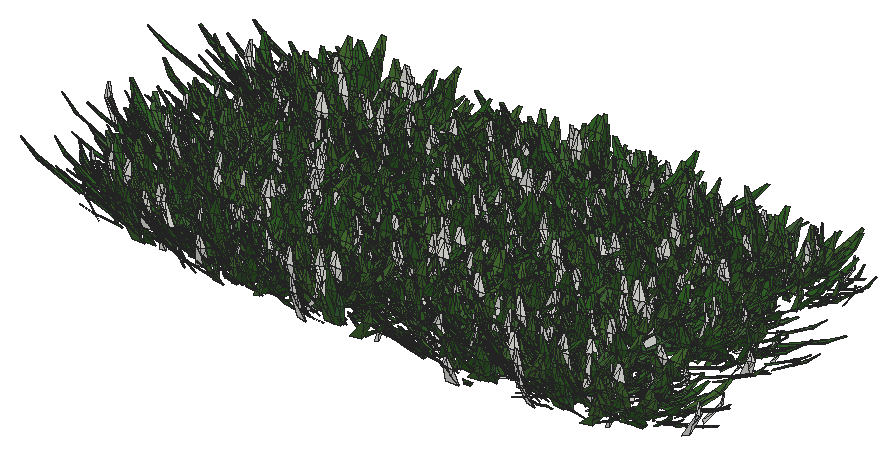
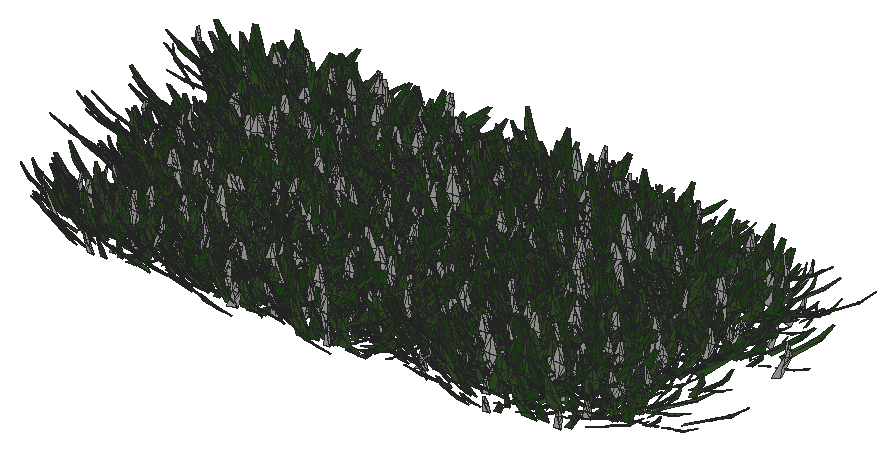
# SketchUp Ruby script. Lengths in inches.
U = 1.inch
M = Sketchup.active_model
def pt(a) = Geom::Point3d.new(a.map { |v| v * U })
def face(e, loops, mat)
  f = e.add_face(loops[0].map { |a| pt(a) })
  loops[1..].each { |l| e.add_face(l.map { |a| pt(a) }).erase! }
  f.material = f.back_material = mat if mat
  f
end
# faces: each face lists its corners as indices into pts; further lists are holes
def faces(e, pts, list, mat = nil) = list.each { |f| face(e, (f[0].is_a?(Array) ? f : [f]).map { |l| l.map { |i| pts[i] } }, mat) }
# xy, xz, yz: faces in a plane at the given z, y or x. An outline is a flat list of corners, or four numbers for a rectangle; further outlines are holes
def ring(l) = l.size == 4 ? [[l[0], l[1]], [l[2], l[1]], [l[2], l[3]], [l[0], l[3]]] : l.each_slice(2).to_a
def flat(e, list, mat, &to3) = list.each { |f| face(e, (f[0].is_a?(Array) ? f : [f]).map { |l| ring(l).map { |u, v| to3.(u, v) } }, mat) }
def xy(e, z, list, mat = nil) = flat(e, list, mat) { |x, y| [x, y, z] }
def xz(e, y, list, mat = nil) = flat(e, list, mat) { |x, z| [x, y, z] }
def yz(e, x, list, mat = nil) = flat(e, list, mat) { |y, z| [x, y, z] }
def lines(e, pts, list) = list.each { |a, b| e.add_line(pt(pts[a]), pt(pts[b])) }
# prism: a flat outline (further loops are holes) pulled along v
def prism(e, loops, v, mat = nil)
  f = face(e, loops, mat); d = Geom::Vector3d.new(v.map { |x| x * U })
  f.pushpull(f.normal.samedirection?(d) ? d.length : -d.length)
end
def box(e, o, s, mat = nil) = prism(e, [[o, [o[0] + s[0], o[1], o[2]], [o[0] + s[0], o[1] + s[1], o[2]], [o[0], o[1] + s[1], o[2]]]], [0, 0, s[2]], mat)
def at(x, y, z, deg = 0) = Geom::Transformation.translation(pt([x, y, z])) * Geom::Transformation.rotation(ORIGIN, Z_AXIS, deg.degrees)
def axes(o, x, y, z) = Geom::Transformation.new([*x, 0, *y, 0, *z, 0, *pt(o).to_a, 1])
def part(name) = M.definitions.add(name)
# library, detail: a bought-in or finely detailed component or shape, given as its bounding box
def library(name, o, s) = part(name).tap { |d| box(d.entities, o, s) }
def detail(e, o, s) = box(e.add_group.entities, o, s)
def put(e, d, t, mat = nil) = e.add_instance(d, t).tap { |i| i.material = mat if mat }
def group(e, t, mat = nil) = e.add_group.tap { |g| g.transformation = t; g.material = mat if mat }.entities
root = M.entities
M.materials.add("Material82").color = [68, 110, 58]
M.materials.add("Material83").color = [48, 90, 38]
M.materials.add("Material84").color = [68, 110, 48]
M.materials.add("Material85").color = [48, 90, 48]
M.materials.add("Material86").color = [58, 110, 58]
M.materials.add("Material87").color = [58, 90, 38]
M.materials.add("Material88").color = [68, 100, 58]
M.materials.add("Material89").color = [48, 100, 38]
c1 = part("grass00")
p = [[-0.6875,0.15,0],[-0.56,0.08,5.52],[-0.04,0.03,2.76],[0.48,-0.02,0],[0.35,-0.02,5.52],[-0.1,-0.14,5.52],
  [-0.12,0.65,8.37],[-0.42,0.65,8.37]]
faces(c1.entities,p,[[0,1,2,3],[3,2,4],[1,5,2],[5,4,2],[1,6,5],[4,5,6],[7,6,1]])
c2 = part("Group16\#1")
put(c2.entities,c1,axes([1.44,-0.61,-0.01],[0.05352,0.12609,0],[-0.10704,0.04543,0.07239],[0.06664,-0.02828,0.11628]),"Material85")
put(c2.entities,c1,axes([0.76,-0.15,-0.01],[0.04676,0.24062,0],[-0.23162,0.04501,0.06642],[0.0652,-0.01267,0.23595]),"Material82")
put(c2.entities,c1,axes([0.79,0.01,-0.01],[-0.00606,0.34651,0],[-0.34381,-0.00602,0.0432],[0.04319,0.00076,0.34386]))
put(c2.entities,c1,axes([1,0.23,-0.01],[-0.07192,0.31144,0],[-0.28722,-0.06632,0.1236],[0.12043,0.02781,0.29478]),"Material84")
put(c2.entities,c1,axes([1.66,0.77,-0.01],[-0.13828,0.29651,0],[-0.21551,-0.1005,0.22471],[0.20365,0.09498,0.23779]),"Material89")
put(c2.entities,c1,axes([0.6875,0.52,-0.01],[-0.18126,0.24051,0],[-0.22746,-0.17142,0.09788],[0.07817,0.05891,0.28481]),"Material84")
put(c2.entities,c1,axes([0.68,0.78,-0.01],[-0.215,0.18688,0],[-0.12385,-0.14248,0.21334],[0.13995,0.16101,0.18878]),"Material82")
put(c2.entities,c1,axes([0.56,1,-0.01],[-0.13756,0.07624,0],[-0.06159,-0.11112,0.0927],[0.04494,0.08108,0.12705]),"Material84")
put(c2.entities,c1,axes([0.2,0.64,-0.01],[-0.23729,0.07254,0],[-0.05711,-0.18681,0.153],[0.04473,0.14632,0.19535]),"Material89")
put(c2.entities,c1,axes([0.0625,0.72,-0.01],[-0.28874,0.02525,0],[-0.02179,-0.24916,0.14647],[0.01276,0.14591,0.25012]),"Material82")
put(c2.entities,c1,axes([-0.08,0.62,-0.01],[-0.34089,-0.04187,0],[0.03255,-0.26504,0.216],[-0.02633,0.21439,0.26703]),"Material89")
put(c2.entities,c1,axes([-0.34,0.98,-0.01],[-0.14314,-0.0493,0],[0.04397,-0.12769,0.06843],[-0.02228,0.0647,0.13505]),"Material89")
put(c2.entities,c1,axes([-0.87,1.45,-0.01],[-0.23488,-0.14114,0],[0.13761,-0.22901,0.06087],[-0.03135,0.05217,0.26717]))
put(c2.entities,c1,axes([-0.72,0.77,-0.01],[-0.14208,-0.13251,0],[0.07209,-0.0773,0.16301],[-0.11118,0.11922,0.1057]),"Material89")
put(c2.entities,c1,axes([-0.62,0.43,-0.01],[-0.14845,-0.21203,0],[0.18654,-0.13061,0.12304],[-0.10079,0.07057,0.22772]),"Material82")
put(c2.entities,c1,axes([-0.68,0.29,-0.01],[-0.13639,-0.32136,0],[0.31723,-0.13464,0.05579],[-0.05136,0.0218,0.34462]),"Material83")
put(c2.entities,c1,axes([-0.64,0.125,-0.01],[-0.0458,-0.23569,0],[0.22124,-0.043,0.08276],[-0.08124,0.01579,0.22538]),"Material86")
put(c2.entities,c1,axes([-1.6,-0.03,-0.01],[0.00576,-0.32897,0],[0.27526,0.00482,0.18018],[-0.18015,-0.00315,0.2753]),"Material84")
put(c2.entities,c1,axes([-1.36,-0.31,-0.01],[0.05718,-0.24765,0],[0.18172,0.04196,0.17267],[-0.16825,-0.03885,0.1865]),"Material89")
put(c2.entities,c1,axes([-1.54,-0.72,-0.01],[0.06537,-0.14017,0],[0.13555,0.06321,0.03939],[-0.0357,-0.01665,0.14956]))
put(c2.entities,c1,axes([-1.19,-0.9,-0.01],[0.09597,-0.12735,0],[0.11214,0.08451,0.07557],[-0.06035,-0.04548,0.14042]),"Material88")
put(c2.entities,c1,axes([-0.47,-0.54,-0.01],[0.11588,-0.10072,0],[0.0618,0.0711,0.12124],[-0.07953,-0.0915,0.0942]))
put(c2.entities,c1,axes([-0.47,-0.84,-0.01],[0.11927,-0.0661,0],[0.06603,0.11913,0.00646],[-0.00313,-0.00565,0.13621]),"Material84")
put(c2.entities,c1,axes([-0.38,-1.24,-0.01],[0.28037,-0.08571,0],[0.0618,0.20215,0.20315],[-0.05939,-0.19428,0.21139]),"Material88")
put(c2.entities,c1,axes([-0.06,-0.66,-0.01],[0.22719,-0.01987,0],[0.01247,0.14255,0.17758],[-0.01547,-0.17691,0.1431]),"Material87")
put(c2.entities,c1,axes([0.11,-0.89,-0.01],[0.14882,0.01828,0],[-0.01058,0.08611,0.12229],[0.01491,-0.12138,0.08676]),"Material85")
put(c2.entities,c1,axes([0.25,-0.72,-0.01],[0.20481,0.07053,0],[-0.06206,0.18022,0.10291],[0.03351,-0.0973,0.1906]),"Material85")
put(c2.entities,c1,axes([0.85,-1.42,-0.01],[0.16481,0.09904,0],[-0.09472,0.15762,0.05616],[0.02893,-0.04814,0.18389]),"Material84")
put(c2.entities,c1,axes([1.01,-1.09,-0.01],[0.21858,0.20385,0],[-0.17495,0.1876,0.15339],[0.10462,-0.11218,0.25652]),"Material89")
put(c2.entities,c1,axes([1.01,-0.71,-0.01],[0.08733,0.12473,0],[-0.06445,0.04512,0.13037],[0.1068,-0.07477,0.07867]),"Material85")
c3 = part("Group15\#1")
put(c3.entities,c2,at(0,0,0))
c4 = part("3darcstudiotree_grass00\#1")
put(c4.entities,c3,at(0,0,0))
put(root,c4,axes([648.16,366.61,-34.17],[-3.83744,0.33373,0],[-0.9251,-1.65441,-0.02531],[-0.02998,-0.05361,1.77094]))
put(root,c4,axes([646.9,353.22,-34.17],[3.34663,1.11106,0],[-2.8307,1.32609,-0.01247],[-0.04541,0.02127,1.86292]))
put(root,c4,axes([649.82,360.98,-34.17],[-3.55958,-1.14913,0],[2.41323,-1.16263,-0.04086],[0.15936,-0.07677,1.75811]))
put(root,c4,axes([650.11,351.33,-34.17],[-0.43927,-1.56699,0],[3.3973,-0.14812,-0.00454],[0.02991,-0.0013,1.6986]))
put(root,c4,axes([650.46,345.77,-34.17],[-1.97176,-1.44506,0],[3.679,-0.78074,-0.04084],[0.18174,-0.03857,1.58232]))
put(root,c4,axes([650.28,344.4375,-34.17],[-3.51315,0.12017,0],[-0.35069,-1.59447,-0.04163],[-0.0224,-0.10183,1.89396]))
put(root,c4,axes([651.03,359.99,-34.17],[-1.25158,-1.24653,0],[3.09013,-0.48255,-0.01359],[0.08484,-0.01325,1.67314]))
put(root,c4,axes([650.44,366.44,-34.17],[-2.97894,1.37787,0],[-2.78264,-0.93567,-0.01811],[-0.06538,-0.02199,1.30017]))
put(root,c4,axes([650.71,354.66,-34.17],[3.2382,0.426,0],[-1.27463,1.50694,-0.00681],[-0.01361,0.01609,1.90695]))
put(root,c4,axes([652.54,370.73,-34.17],[0.12202,-1.72029,0],[4.34373,0.04792,-0.00421],[0.02346,0.00026,1.81536]))
put(root,c4,axes([651.02,352.6875,-34.17],[3.02682,0.57541,0],[-1.48298,1.21327,-0.04063],[-0.10557,0.08637,1.53169]))
put(root,c4,axes([651.15,347.92,-34.17],[-0.79088,1.37944,0],[-4.55872,-0.4065,-0.04071],[-0.16308,-0.01454,1.43871]))
put(root,c4,axes([653.47,368.09,-34.17],[1.28722,-1.76401,0],[4.46987,0.50729,-0.04991],[0.26732,0.03034,1.94306]))
put(root,c4,axes([652.59,357.65,-34.17],[3.67827,0.2088,0],[-0.57305,1.57009,-0.04848],[-0.0346,0.09479,1.51023]))
put(root,c4,axes([653.69,364.37,-34.17],[1.80491,-1.57701,0],[4.14536,0.7379,-0.03311],[0.16907,0.03009,1.9099]))
put(root,c4,axes([653.62,341.82,-34.17],[-0.04598,1.31401,0],[-3.68449,-0.02005,-0.02407],[-0.13013,-0.00071,1.49365]))
put(root,c4,axes([656.17,349.01,-34.17],[0.08239,-1.33128,0],[3.65037,0.03514,-0.00377],[0.02295,0.00022,1.66719]))
put(root,c4,axes([655.74,367.54,-34.17],[-1.91663,1.65988,0],[-3.0087,-0.54032,-0.04508],[-0.21948,-0.03942,1.32557]))
put(root,c4,axes([655.92,357.93,-34.17],[-2.0309,1.41107,0],[-3.96455,-0.88745,-0.03094],[-0.10652,-0.02384,1.35284]))
put(root,c4,axes([655.73,359.23,-34.17],[3.97679,-0.10087,0],[0.2922,1.7917,-0.04097],[0.01281,0.07857,1.66267]))
put(root,c4,axes([656.4,365.41,-34.17],[2.96266,-0.9536,0],[2.21709,1.07131,-0.03627],[0.16479,0.07963,1.88825]))
put(root,c4,axes([657.56,350.52,-34.17],[-2.64678,-1.36079,0],[3.05956,-0.92555,-0.03114],[0.16031,-0.04849,1.87535]))
put(root,c4,axes([656.09,353.46,-34.17],[1.36747,1.27936,0],[-3.91602,0.651,-0.04214],[-0.23603,0.03924,1.93625]))
put(root,c4,axes([657.96,372.32,-34.17],[-0.46652,-1.63259,0],[3.80254,-0.169,-0.02839],[0.12966,-0.00576,1.31807]))
put(root,c4,axes([657.77,362.02,-34.17],[-2.52022,1.35688,0],[-2.71694,-0.78485,-0.02032],[-0.10759,-0.03108,1.65635]))
put(root,c4,axes([658.41,342.15,-34.17],[-3.93546,0.24929,0],[-0.63824,-1.56709,-0.04907],[-0.04216,-0.10352,1.63442]))
put(root,c4,axes([657.29,363.85,-34.17],[0.89151,1.73156,0],[-4.53511,0.36315,-0.02679],[-0.1364,0.01092,1.80175]))
put(root,c4,axes([657.875,343.8125,-34.17],[3.29656,-0.16392,0],[0.52833,1.6525,-0.05027],[0.03097,0.09687,1.55905]))
put(root,c4,axes([658.72,355.55,-34.17],[2.92684,-0.73502,0],[1.91435,1.18558,-0.0345],[0.12831,0.07947,1.8497]))
put(root,c4,axes([658.91,346.87,-34.17],[0.10092,1.39888,0],[-4.08431,0.04583,-0.02239],[-0.13434,0.00151,1.83839]))
put(root,c4,axes([658.99,370.06,-34.17],[-0.46714,1.44095,0],[-4.49775,-0.22678,-0.0277],[-0.15196,-0.00766,1.87956]))
put(root,c4,axes([661.02,360.11,-34.17],[-2.63576,-1.28026,0],[3.53005,-1.13032,-0.02494],[0.11128,-0.03563,1.95866]))
put(root,c4,axes([660.72,370.33,-34.17],[-0.06008,-1.38054,0],[4.09358,-0.02771,-0.0405],[0.24938,-0.00169,1.89003]))
put(root,c4,axes([661.88,362.39,-34.17],[-2.86404,-0.64452,0],[1.81455,-1.25407,-0.04344],[0.15373,-0.10625,1.9596]))
put(root,c4,axes([662.12,350.28,-34.17],[-1.66133,-1.5225,0],[4.09169,-0.6944,-0.04688],[0.21591,-0.03664,1.67419]))
put(root,c4,axes([662.05,356.79,-34.17],[-3.61877,0.99301,0],[-2.17277,-1.23149,-0.01001],[-0.02667,-0.01512,1.32974]))
put(root,c4,axes([663.0625,368.29,-34.17],[-0.34586,-1.45501,0],[4.09876,-0.15153,-0.00863],[0.04038,-0.00149,1.44957]))
put(root,c4,axes([663.64,355.14,-34.17],[-1.55676,-1.64059,0],[4.33421,-0.63965,-0.05081],[0.20494,-0.03024,1.49393]))
put(root,c4,axes([662.23,365.77,-34.17],[4.37611,-0.60729,0],[1.31361,1.47222,-0.0057],[0.0109,0.01221,1.70987]))
put(root,c4,axes([664.14,343.71,-34.17],[-3.927,-0.17218,0],[0.45946,-1.62986,-0.05312],[0.03146,-0.11159,1.67036]))
put(root,c4,axes([663.05,341.7,-34.17],[4.2823,-0.66393,0],[1.32307,1.32724,-0.00849],[0.02062,0.02068,1.79934]))
put(root,c4,axes([664.36,363.99,-34.17],[-3.78815,1.05417,0],[-2.08305,-1.1642,0],[-0.00001,-0.00001,1.91868]))
put(root,c4,axes([663.62,340.27,-34.17],[3.14187,0.39177,0],[-1.17778,1.46906,-0.04459],[-0.07661,0.09555,1.66873]))
put(root,c4,axes([664.52,346.79,-34.17],[-2.14427,1.00131,0],[-3.09998,-1.03248,-0.03207],[-0.1604,-0.05342,1.99077]))
put(root,c4,axes([664.71,348.81,-34.17],[-3.03453,1.36043,0],[-3.50876,-1.21725,-0.06393],[-0.1925,-0.06678,1.40472]))
put(root,c4,axes([664.53,352.39,-34.17],[4.55933,-0.17295,0],[0.45061,1.84755,-0.06081],[0.02387,0.09789,1.44654]))
put(root,c4,axes([666.4,367.64,-34.17],[-0.03672,-1.35909,0],[4.67682,-0.01965,-0.05216],[0.20276,-0.00085,1.36288]))
put(root,c4,axes([666.5,353.11,-34.17],[0.13892,-1.80916,0],[4.0915,0.04886,-0.01983],[0.09749,0.00116,1.50947]))
put(root,c4,axes([666.9,357.1,-34.17],[-3.75519,-1.14447,0],[2.68213,-1.36874,-0.06061],[0.1619,-0.08262,1.43628]))
put(root,c4,axes([666.42,369.82,-34.17],[-0.54027,-1.6401,0],[3.32557,-0.17038,-0.04034],[0.23473,-0.01203,1.47504]))
put(root,c4,axes([666.66,365.63,-34.17],[-3.58356,0.46021,0],[-1.0679,-1.2933,-0.04555],[-0.08783,-0.10637,1.60995]))
put(root,c4,axes([667.12,343.83,-34.17],[-3.8661,0.57248,0],[-1.34665,-1.41442,-0.01194],[-0.02505,-0.02631,1.71307]))
put(root,c4,axes([667.32,351.27,-34.17],[-3.59396,1.08002,0],[-2.30452,-1.19271,-0.04347],[-0.15376,-0.07958,1.66314]))
put(root,c4,axes([668.11,340.48,-34.17],[-3.24117,-0.71309,0],[1.62667,-1.14993,-0.00653],[0.01841,-0.01301,1.4475]))
put(root,c4,axes([666.82,363.49,-34.17],[-0.46786,1.28327,0],[-3.81344,-0.21623,-0.00494],[-0.02392,-0.00136,1.4129]))
put(root,c4,axes([668.61,346.46,-34.17],[0.52643,-1.67667,0],[4.29673,0.20982,-0.00236],[0.01155,0.00056,1.5989]))
put(root,c4,axes([667.55,348.07,-34.17],[4.26757,-0.1267,0],[0.26808,1.40432,-0.02417],[0.01226,0.06424,1.80918]))
put(root,c4,axes([669.16,359.21,-34.17],[-4.03193,0.12785,0],[-0.33897,-1.66251,-0.04274],[-0.01416,-0.06944,1.31001]))
put(root,c4,axes([667.79,361.24,-34.17],[2.51292,1.08795,0],[-3.26468,1.1728,-0.05824],[-0.20485,0.07359,1.57486]))
put(root,c4,axes([668.28,341.95,-34.17],[2.57949,0.81299,0],[-2.19489,1.0831,-0.04441],[-0.18645,0.09201,1.772]))
put(root,c4,axes([669.45,354.82,-34.17],[1.65411,1.32331,0],[-4.02119,0.78176,-0.01549],[-0.05875,0.01142,1.42146]))
put(root,c4,axes([672.18,341.48,-34.17],[-1.99996,-1.21087,0],[3.64955,-0.93751,-0.00487],[0.02184,-0.00561,1.74651]))
put(root,c4,axes([672.43,344.25,-34.17],[0.76825,-1.34447,0],[4.07723,0.36235,-0.02216],[0.10533,0.00936,1.52603]))
put(root,c4,axes([673.35,353.16,-34.17],[-0.47602,-1.5827,0],[4.1601,-0.1946,-0.02638],[0.12052,-0.00564,1.44452]))
put(root,c4,axes([672.65,361.75,-34.17],[-1.67139,1.30839,0],[-3.46219,-0.68786,-0.03585],[-0.17478,-0.03472,1.58646]))
put(root,c4,axes([673.24,368.33,-34.17],[-3.50073,0.942,0],[-2.16331,-1.25037,-0.04776],[-0.1565,-0.09046,1.6727]))
put(root,c4,axes([672.59,360.04,-34.17],[3.80678,-0.63656,0],[1.53404,1.42681,-0.02583],[0.05775,0.05372,1.68703]))
put(root,c4,axes([673.54,354.56,-34.17],[3.46257,-0.87441,0],[2.25752,1.39035,-0.00312],[0.00811,0.00499,1.51309]))
put(root,c4,axes([673.17,357.61,-34.17],[4.45522,-0.42871,0],[0.88291,1.42703,-0.01844],[0.02851,0.04608,1.82062]))
put(root,c4,axes([674.21,348.22,-34.17],[2.70908,-1.29001,0],[3.26836,1.0675,-0.01649],[0.07179,0.02345,1.79785]))
put(root,c4,axes([674.9375,370.96,-34.17],[-1.99014,-1.36063,0],[3.61455,-0.82226,-0.05686],[0.20653,-0.04698,1.31145]))
put(root,c4,axes([674.6,366.26,-34.17],[1.2093,-1.57862,0],[4.10109,0.48862,-0.03916],[0.21176,0.02523,1.81408]))
put(root,c4,axes([673.14,372.33,-34.17],[2.22707,1.32751,0],[-3.83725,1.00121,-0.02773],[-0.10131,0.02643,1.51065]))
put(root,c4,axes([674.125,345.68,-34.17],[3.29328,0.79365,0],[-2.38723,1.54066,-0.04231],[-0.12354,0.07973,1.92144]))
put(root,c4,axes([675.84,351.2,-34.17],[-4.33123,0.18779,0],[-0.372,-1.33439,-0.04038],[-0.02759,-0.09898,1.5952]))
put(root,c4,axes([675.48,340.03,-34.17],[-2.43738,1.19248,0],[-2.72185,-0.86527,-0.02131],[-0.12,-0.03815,1.8955]))
put(root,c4,axes([675.43,364.4,-34.17],[-1.08989,1.28976,0],[-3.11811,-0.40981,-0.02384],[-0.1661,-0.02183,1.80943]))
put(root,c4,axes([677.33,372.52,-34.17],[0.31301,-1.31124,0],[3.5948,0.13346,-0.01523],[0.11152,0.00414,1.99019]))
put(root,c4,axes([677.89,345.68,-34.17],[-3.40339,-1.11564,0],[2.13204,-1.01156,-0.01701],[0.08509,-0.04037,1.95649]))
put(root,c4,axes([678.25,358.8125,-34.17],[-3.55731,-0.39699,0],[0.91028,-1.26863,-0.03071],[0.04629,-0.06451,1.38702]))
put(root,c4,axes([677.75,353.5,-34.17],[1.53941,-1.17663,0],[3.76142,0.76538,-0.04957],[0.23972,0.04878,1.72633]))
put(root,c4,axes([677.95,351.05,-34.17],[1.91221,-1.68967,0],[4.00415,0.70478,-0.04062],[0.20203,0.03556,1.79015]))
put(root,c4,axes([677.82,357.86,-34.17],[3.14616,-0.46124,0],[1.36147,1.44435,-0.02775],[0.06352,0.06739,1.92398]))
put(root,c4,axes([679.21,366.51,-34.17],[-0.59398,-1.49967,0],[3.68059,-0.22673,-0.04759],[0.22724,-0.014,1.34947]))
put(root,c4,axes([680.06,355.07,-34.17],[1.44153,-1.60776,0],[3.23959,0.45176,-0.02361],[0.11408,0.01591,1.32009]))
put(root,c4,axes([679.49,349.43,-34.17],[-0.86085,1.83609,0],[-4.61027,-0.33618,-0.00297],[-0.01572,-0.00115,1.8915]))
put(root,c4,axes([679.41,342.07,-34.17],[2.91821,1.08875,0],[-2.82314,1.17688,-0.00432],[-0.01382,0.00576,1.43292]))
put(root,c4,axes([680.67,370.32,-34.17],[3.48292,-0.82099,0],[2.25154,1.48559,-0.05659],[0.14545,0.09597,1.64805]))
put(root,c4,axes([680.1,368.5,-34.17],[3.42406,1.01361,0],[-2.506,1.31662,-0.02233],[-0.08435,0.04432,1.9689]))
put(root,c4,axes([680.82,361.89,-34.17],[-2.64058,1.54622,0],[-3.55505,-0.94424,-0.0002],[-0.001,-0.00026,1.96126]))
put(root,c4,axes([681.16,363.25,-34.17],[4.33275,-0.34682,0],[0.77843,1.5125,-0.04034],[0.04996,0.09707,1.82611]))
put(root,c4,axes([681.125,345.04,-34.17],[3.65442,0.79234,0],[-1.92667,1.38205,-0.0244],[-0.05154,0.03697,1.31386]))
put(root,c4,axes([683.54,364.07,-34.17],[-4.47242,-0.43212,0],[1.12449,-1.81009,-0.038],[0.04833,-0.0778,1.89315]))
put(root,c4,axes([684.62,357.43,-34.17],[2.42149,-1.19086,0],[3.28427,1.03866,-0.04277],[0.16953,0.05361,1.60323]))
put(root,c4,axes([685.58,346.67,-34.17],[-4.5051,-0.1347,0],[0.33952,-1.76605,-0.05601],[0.0175,-0.09103,1.39118]))
put(root,c4,axes([685.71,350.83,-34.17],[-3.05686,-1.19982,0],[3.00062,-1.189,-0.05331],[0.20258,-0.08027,1.71744]))
put(root,c4,axes([685.7,348.13,-34.17],[0.58993,-1.49665,0],[4.0908,0.25078,-0.01704],[0.09795,0.00601,1.80481]))
put(root,c4,axes([684.26,343.77,-34.17],[0.93986,1.81776,0],[-4.11362,0.3308,-0.03996],[-0.17618,0.01417,1.416]))
put(root,c4,axes([684.26,372.17,-34.17],[1.86,1.67689,0],[-3.22779,0.55683,-0.02724],[-0.14202,0.0245,1.50258]))
put(root,c4,axes([684.55,355.82,-34.17],[3.80375,0.01195,0],[-0.02861,1.41659,-0.01492],[-0.00081,0.04025,1.84219]))
put(root,c4,axes([685.61,365.9375,-34.17],[-1.91722,1.31385,0],[-4.0358,-0.91594,-0.03664],[-0.12047,-0.02734,1.3241]))
put(root,c4,axes([685.85,359.45,-34.17],[4.38931,-0.45982,0],[1.18067,1.75286,-0.06211],[0.07411,0.11002,1.60192]))
put(root,c4,axes([685.58,371.3,-34.17],[3.90875,0.99817,0],[-2.33451,1.4218,-0.02279],[-0.07245,0.04412,1.88252]))
put(root,c4,axes([686.16,361.58,-34.17],[4.17909,0.84834,0],[-2.02565,1.55199,-0.04224],[-0.09233,0.07074,1.58426]))
put(root,c4,axes([686.57,341.35,-34.17],[3.56991,0.07978,0],[-0.21949,1.52742,-0.02759],[-0.00848,0.05902,1.57942]))
put(root,c4,axes([688.38,354.51,-34.17],[-4.32084,-0.18562,0],[0.42888,-1.55273,-0.0047],[0.00255,-0.00922,1.4854]))
put(root,c4,axes([686.82,368.89,-34.17],[0.16976,1.81896,0],[-4.60297,0.06681,-0.03073],[-0.13236,0.00192,1.48809]))
put(root,c4,axes([688.74,371.02,-34.17],[-3.5417,-0.59044,0],[1.62012,-1.51145,-0.0473],[0.08471,-0.07903,1.43445]))
put(root,c4,axes([686.9375,353.31,-34.17],[4.0668,0.76332,0],[-1.54133,1.27718,-0.01473],[-0.03515,0.02913,1.49308]))
put(root,c4,axes([688.53,357.81,-34.17],[-3.98791,0.79031,0],[-1.65069,-1.29546,-0.0516],[-0.1637,-0.12847,1.94674]))
put(root,c4,axes([689.05,361.73,-34.17],[-3.83726,0.13979,0],[-0.31883,-1.36117,-0.04806],[-0.027,-0.11528,1.58689]))
put(root,c4,axes([689.89,350.08,-34.17],[-3.41944,0.15794,0],[-0.40533,-1.36487,-0.03745],[-0.0251,-0.08453,1.50509]))
put(root,c4,axes([688.6,344.37,-34.17],[0.51016,1.70246,0],[-4.00788,0.18679,-0.00527],[-0.02601,0.00121,1.50433]))
put(root,c4,axes([689.07,372.3,-34.17],[3.76255,0.21279,0],[-0.50611,1.39184,-0.02285],[-0.01632,0.04489,1.34478]))
put(root,c4,axes([690.53,340.09,-34.17],[-4.15336,0.88478,0],[-2.07336,-1.51373,-0.03525],[-0.06704,-0.04895,1.3087]))
put(root,c4,axes([690.7,347.01,-34.17],[1.23783,-1.57966,0],[3.18362,0.388,-0.00928],[0.06663,0.00812,1.87692]))
put(root,c4,axes([689.54,359.74,-34.17],[4.18297,0.824,0],[-1.87304,1.47883,-0.04234],[-0.08644,0.06825,1.4356]))
put(root,c4,axes([692.39,367.52,-34.17],[-4.24589,-0.20577,0],[0.52914,-1.69815,-0.04768],[0.02678,-0.08595,1.49744]))
put(root,c4,axes([690.91,352.74,-34.17],[0.88024,1.52698,0],[-4.39329,0.39388,-0.06457],[-0.26955,0.02417,1.44574]))
put(root,c4,axes([691.93,341.93,-34.17],[2.74133,-1.23391,0],[3.31507,1.14547,-0.04981],[0.18948,0.06547,1.67091]))
put(root,c4,axes([691.04,365.63,-34.17],[3.13752,1.05459,0],[-2.29496,1.06192,-0.00613],[-0.02513,0.01163,1.67562]))
put(root,c4,axes([691.9,347.84,-34.17],[1.5924,1.20755,0],[-3.44476,0.70651,-0.03549],[-0.1652,0.03388,1.52707]))
put(root,c4,axes([691.68,364.09,-34.17],[1.54833,1.52017,0],[-4.09421,0.64856,-0.00669],[-0.03642,0.00577,1.94122]))
put(root,c4,axes([694.36,363.53,-34.17],[-0.04856,-1.33378,0],[4.56796,-0.02587,-0.06189],[0.3016,-0.00171,1.66883]))
put(root,c4,axes([695.58,370.44,-34.17],[-4.54384,0.18076,0],[-0.35947,-1.40543,-0.00469],[-0.00344,-0.01343,1.96044]))
put(root,c4,axes([695.93,342.31,-34.17],[-3.26554,0.66263,0],[-1.53451,-1.17616,-0.01759],[-0.06154,-0.04717,1.92222]))
put(root,c4,axes([695.71,354.88,-34.17],[2.51439,-1.31879,0],[3.78,1.12088,-0.05965],[0.2657,0.07879,1.97549]))
put(root,c4,axes([696.5,356.6,-34.17],[-0.70547,-1.57622,0],[3.40493,-0.23702,-0.01992],[0.12135,-0.00845,1.60321]))
put(root,c4,axes([694.93,350.71,-34.17],[4.47557,0.19067,0],[-0.50576,1.84642,-0.03307],[-0.01603,0.05854,1.59331]))
put(root,c4,axes([695.36,366.21,-34.17],[0.58274,1.76141,0],[-3.38049,0.17394,-0.03746],[-0.24477,0.01259,1.68385]))
put(root,c4,axes([696.04,347.91,-34.17],[-3.09447,0.74267,0],[-2.17746,-1.41107,-0.01391],[-0.03982,-0.0258,1.7292]))
put(root,c4,axes([696.26,352.47,-34.17],[2.464,-1.39681,0],[2.85004,0.78193,-0.02795],[0.16419,0.04505,1.86246]))
put(root,c4,axes([696.15,359.98,-34.17],[-1.84293,1.54258,0],[-3.69335,-0.68627,-0.00165],[-0.00726,-0.00135,1.48801]))
put(root,c4,axes([697.75,343.68,-34.17],[-4.60496,-0.17881,0],[0.42059,-1.68464,-0.00134],[0.00055,-0.00219,1.33719]))
put(root,c4,axes([697.33,346.44,-34.17],[2.67997,-1.42027,0],[3.59345,1.05458,-0.05496],[0.18586,0.05455,1.41537]))
put(root,c4,axes([697.52,361.42,-34.17],[0.63899,1.37464,0],[-4.27438,0.30902,-0.00804],[-0.04314,0.00312,1.77733]))
put(root,c4,axes([697.76,368.8,-34.17],[1.87438,1.56788,0],[-3.52749,0.65588,-0.03917],[-0.21764,0.04047,1.79585]))
put(root,c4,axes([700.28,343.99,-34.17],[-1.02752,-1.39563,0],[3.42384,-0.39205,-0.00444],[0.02976,-0.00341,1.86591]))
put(root,c4,axes([699.71,363.61,-34.17],[1.33366,-1.36849,0],[3.54112,0.53673,-0.03841],[0.22056,0.03343,1.74904]))
put(root,c4,axes([700.18,372.1875,-34.17],[-1.96103,-1.06216,0],[3.43549,-0.98649,-0.06067],[0.27868,-0.08002,1.80988]))
put(root,c4,axes([700.07,348.42,-34.17],[-3.04968,0.59415,0],[-1.75652,-1.40223,-0.03032],[-0.06781,-0.05413,1.50108]))
put(root,c4,axes([700.65,340.7,-34.17],[-2.6125,1.23987,0],[-2.75746,-0.90365,-0.04997],[-0.20997,-0.06881,1.46822]))
put(root,c4,axes([700.38,347,-34.17],[-0.25979,1.36498,0],[-3.68566,-0.1091,-0.02554],[-0.15097,-0.00447,1.64241]))
put(root,c4,axes([702.14,352.27,-34.17],[-4.34871,0.30764,0],[-0.79873,-1.75601,-0.00093],[-0.00077,-0.00169,1.58752]))
put(root,c4,axes([700.95,342.48,-34.17],[3.80887,0.06416,0],[-0.18164,1.67717,-0.01987],[-0.00391,0.03608,1.47043]))
put(root,c4,axes([700.98,355.03,-34.17],[4.17174,-0.07865,0],[0.15922,1.3134,-0.03217],[0.01066,0.0879,1.73328]))
put(root,c4,axes([701.18,357.09,-34.17],[3.86863,-0.34225,0],[0.73265,1.28801,-0.00297],[0.00437,0.00768,1.68702]))
put(root,c4,axes([701.38,366.9,-34.17],[3.26947,0.70015,0],[-1.66816,1.21153,-0.03457],[-0.12105,0.08791,1.92264]))
put(root,c4,axes([701.95,351.22,-34.17],[-1.46805,1.46647,0],[-4.14161,-0.64484,-0.02576],[-0.10998,-0.01712,1.53201]))
put(root,c4,axes([702.03,359.15,-34.17],[4.25624,-0.01859,0],[0.03959,1.4097,-0.01976],[0.00112,0.03979,1.36845]))
put(root,c4,axes([702.26,370.34,-34.17],[2.49415,0.97261,0],[-2.31115,0.92177,-0.02576],[-0.13853,0.05525,1.88472]))
put(root,c4,axes([703.48,360.97,-34.17],[-2.30622,1.23379,0],[-2.8482,-0.82802,-0.0238],[-0.11552,-0.03358,1.59896]))
put(root,c4,axes([703.11,369.02,-34.17],[1.30118,1.34593,0],[-3.49846,0.52602,-0.01397],[-0.0708,0.01064,1.52193]))
put(root,c4,axes([705.68,342.78,-34.17],[-2.87014,-1.48867,0],[3.23188,-0.96911,-0.02],[0.09309,-0.02792,1.779]))
put(root,c4,axes([705.46,344.18,-34.17],[-0.3493,-1.81077,0],[4.63308,-0.139,-0.05882],[0.26935,-0.00808,1.5994]))
put(root,c4,axes([705.83,355.86,-34.17],[-3.58056,-0.39826,0],[0.95821,-1.33984,-0.015],[0.02011,-0.02812,1.30652]))
